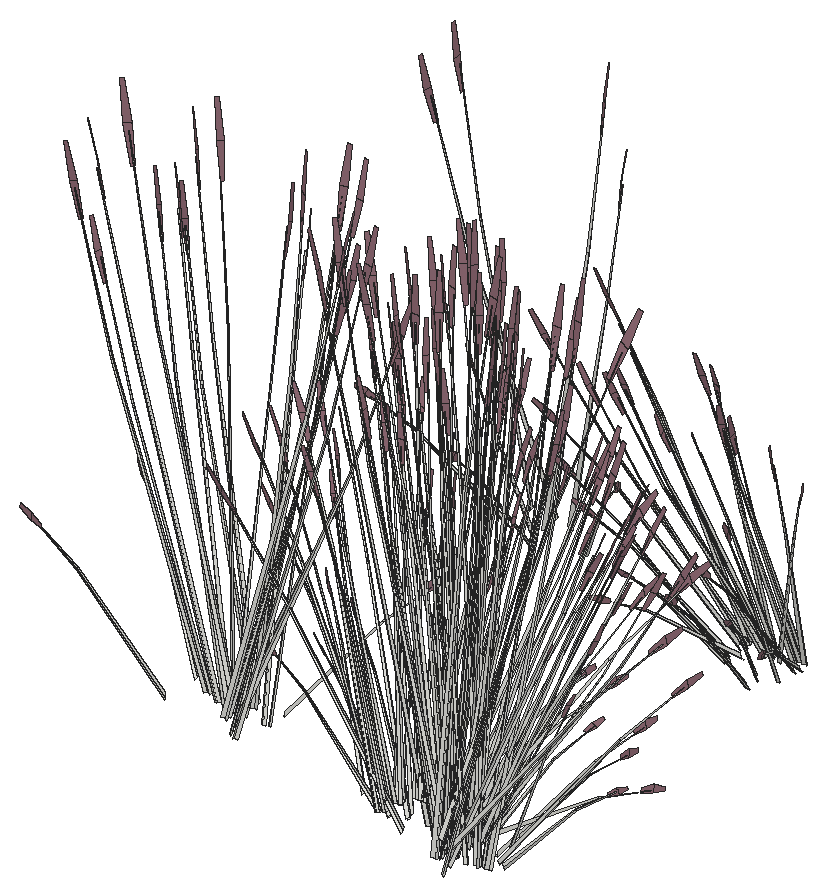
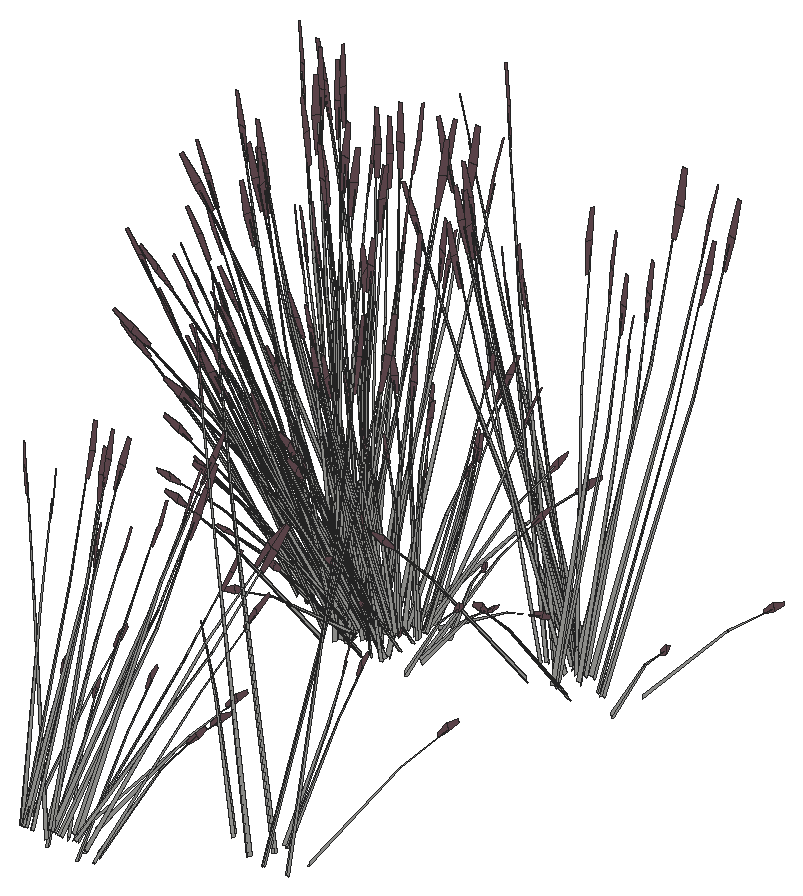
# SketchUp Ruby script. Lengths in inches.
U = 1.inch
M = Sketchup.active_model
def pt(a) = Geom::Point3d.new(a.map { |v| v * U })
def face(e, loops, mat)
  f = e.add_face(loops[0].map { |a| pt(a) })
  loops[1..].each { |l| e.add_face(l.map { |a| pt(a) }).erase! }
  f.material = f.back_material = mat if mat
  f
end
# faces: each face lists its corners as indices into pts; further lists are holes
def faces(e, pts, list, mat = nil) = list.each { |f| face(e, (f[0].is_a?(Array) ? f : [f]).map { |l| l.map { |i| pts[i] } }, mat) }
# xy, xz, yz: faces in a plane at the given z, y or x. An outline is a flat list of corners, or four numbers for a rectangle; further outlines are holes
def ring(l) = l.size == 4 ? [[l[0], l[1]], [l[2], l[1]], [l[2], l[3]], [l[0], l[3]]] : l.each_slice(2).to_a
def flat(e, list, mat, &to3) = list.each { |f| face(e, (f[0].is_a?(Array) ? f : [f]).map { |l| ring(l).map { |u, v| to3.(u, v) } }, mat) }
def xy(e, z, list, mat = nil) = flat(e, list, mat) { |x, y| [x, y, z] }
def xz(e, y, list, mat = nil) = flat(e, list, mat) { |x, z| [x, y, z] }
def yz(e, x, list, mat = nil) = flat(e, list, mat) { |y, z| [x, y, z] }
def lines(e, pts, list) = list.each { |a, b| e.add_line(pt(pts[a]), pt(pts[b])) }
# prism: a flat outline (further loops are holes) pulled along v
def prism(e, loops, v, mat = nil)
  f = face(e, loops, mat); d = Geom::Vector3d.new(v.map { |x| x * U })
  f.pushpull(f.normal.samedirection?(d) ? d.length : -d.length)
end
def box(e, o, s, mat = nil) = prism(e, [[o, [o[0] + s[0], o[1], o[2]], [o[0] + s[0], o[1] + s[1], o[2]], [o[0], o[1] + s[1], o[2]]]], [0, 0, s[2]], mat)
def at(x, y, z, deg = 0) = Geom::Transformation.translation(pt([x, y, z])) * Geom::Transformation.rotation(ORIGIN, Z_AXIS, deg.degrees)
def axes(o, x, y, z) = Geom::Transformation.new([*x, 0, *y, 0, *z, 0, *pt(o).to_a, 1])
def part(name) = M.definitions.add(name)
# library, detail: a bought-in or finely detailed component or shape, given as its bounding box
def library(name, o, s) = part(name).tap { |d| box(d.entities, o, s) }
def detail(e, o, s) = box(e.add_group.entities, o, s)
def put(e, d, t, mat = nil) = e.add_instance(d, t).tap { |i| i.material = mat if mat }
def group(e, t, mat = nil) = e.add_group.tap { |g| g.transformation = t; g.material = mat if mat }.entities
root = M.entities
M.materials.add("LightPink_Translucent").color = [144, 107, 117]
c1 = part("blade")
p = [[2.15,0.21,22],[0,0.17,0],[0.09,0.45,0],[2.18,0.31,22],[2.29,0.31,22],[0.38,0.45,0],
  [2.48,0.24,33],[2.49,0.24,33],[2.48,0.22,33]]
faces(c1.entities,p,[[0,1,2,3],[4,5,2,3],[6,3,4,7],[8,0,3,6]])
c2 = part("seeds")
p = [[0.3,-0.1,1.38],[-0.01,-0.03,1.59],[-0.01,-0.03,0.03],[0.14,-0.07,-0.07],[0.29,-0.03,3],[0.15,0.01,3.11]]
faces(c2.entities,p,[[0,1,2,3],[1,0,4,5]],"LightPink_Translucent")
c3 = part("blade with seeds")
put(c3.entities,c1,at(0,0,0))
put(c3.entities,c2,axes([2.4,0.25,30.99],[1.5799,-0.05474,1.17369],[-0.12525,1.92788,0.29478],[-0.07173,-0.02425,1.56792]))
put(root,c3,axes([43.62,594.39,43.49],[0.03108,0.16322,1.76342],[-0.62654,0.85237,-0.26939],[-0.44504,-0.04296,0.30037]))
put(root,c3,axes([78.5,593.11,40.8125],[-0.50831,0.02346,1.71376],[0.33721,-1.01661,0.13857],[0.72439,0.06288,0.73262]))
put(root,c3,axes([79.16,590.9,38.96],[0.28787,0.90242,-0.30978],[-1.14332,0.25625,0.30978],[0.23049,0.10406,1.38974]))
put(root,c3,axes([46.37,597.46,44.03],[-0.28787,-0.90242,-0.30978],[1.14332,-0.25625,0.30978],[-0.23049,-0.10406,1.38974]))
put(root,c3,axes([81.125,594.51,41.67],[0.4501,0.70615,0.0643],[-0.82077,0.34564,0.50621],[0.36181,-0.0682,0.77189]))
put(root,c3,axes([76.86,592.92,39.32],[-1.54892,-0.2182,0.49198],[0.31522,-1.23236,0.19306],[0.22636,0.119,1.70813]))
put(root,c3,axes([81.04,594.26,41.67],[-0.34623,0.9443,0.48003],[-1.13828,-0.3229,0.3958],[0.44763,-0.05675,0.9933]))
put(root,c3,axes([50.55,593.55,44.67],[1.23732,-0.68758,-0.29095],[0.8228,0.97154,-0.50002],[0.30528,0.09867,1.59708]))
put(root,c3,axes([75.62,595.96,39.14],[-0.39985,-0.89288,0],[1.1418,-0.31268,0],[0,0,1.54371]))
put(root,c3,axes([74.86,595.11,39.55],[-0.23642,0.92427,0.1448],[-1.15506,-0.16044,-0.41347],[-0.21021,-0.09491,1.26744]))
put(root,c3,axes([70.38,592.72,41.99],[1.01846,0.28891,0.35414],[-0.29705,0.84289,-0.4572],[-0.41005,0.07729,0.87481]))
put(root,c3,axes([46.05,597.85,44.02],[-1.14694,-0.51783,-0.49651],[0.68554,-0.92854,0],[-0.26122,-0.11794,1.57504]))
put(root,c3,axes([53.67,591.72,44.02],[1.14694,0.51783,-0.49651],[-0.68554,0.92854,0],[0.26122,0.11794,1.57504]))
put(root,c3,axes([77.12,595.84,39.12],[1.2866,-0.3514,-0.19198],[0.45209,1.01223,0.00008],[0.14202,-0.03884,1.73897]))
put(root,c3,axes([77.5625,596.26,39.41],[0.35402,-1.02926,0.17642],[1.29548,0.29127,0.35086],[-0.22379,0.00501,1.60407]))
put(root,c3,axes([77.27,593.92,39.15],[0.85545,0.66896,0],[-0.85545,0.66896,0],[0,0,1.69266]))
put(root,c3,axes([49.17,596.02,44.67],[-1.23732,0.68758,-0.29095],[-0.8228,-0.97154,-0.50002],[-0.30528,-0.09867,1.59708]))
put(root,c3,axes([72.41,592.67,40.28],[0.34834,-0.14982,1.77064],[0.12012,1.04605,0.13857],[-0.75452,0.1388,0.63284]))
put(root,c3,axes([79.59,593.63,39.41],[-0.96285,-0.75439,0.17642],[0.97031,-0.7317,0.35086],[-0.10634,0.15406,1.60407]))
put(root,c3,axes([77.8,592.49,38.99],[1.27479,0.1698,-0.62353],[-0.26901,1.04736,-0.16365],[0.38043,0.12691,1.37633]))
put(root,c3,axes([83.4375,594.32,39.7],[-0.75718,0.17097,1.1486],[0.35641,-0.70661,0.84392],[0.40168,0.04835,0.25299]))
put(root,c3,axes([53.35,592.11,44.03],[0.28787,0.90242,-0.30978],[-1.14332,0.25625,0.30978],[0.23049,0.10406,1.38974]))
put(root,c3,axes([75.34,596.37,39.13],[-1.23546,-0.46496,0],[0.59459,-0.96613,0],[0,0,1.62707]))
put(root,c3,axes([76.37,595.13,39.4],[-1.19666,-0.83357,-0.25192],[1.00694,-0.93603,0.5513],[-0.32224,0.09751,1.68216]))
put(root,c3,axes([73.22,596.72,39.41],[1.14694,0.51783,0.49651],[-0.68554,0.92854,0],[-0.26122,-0.11794,1.57504]))
put(root,c3,axes([77.26,593.14,39.65],[0.59459,-0.93321,0.44739],[1.23546,0.44912,-0.21531],[0,0.21512,1.43643]))
put(root,c3,axes([83.08,597.3125,41.64],[-0.11081,-0.09067,1.77383],[0.2424,-0.97188,-0.16761],[0.43649,-0.06209,0.31391]))
put(root,c3,axes([51.31,597.04,44.18],[1.2866,-0.3514,-0.19198],[0.45209,1.01223,0.00008],[0.14202,-0.03884,1.73897]))
put(root,c3,axes([68.66,593.37,41.65],[-0.20012,0.13446,1.74944],[0.01702,0.98243,-0.27667],[-0.45871,0.12776,0.14031]))
put(root,c3,axes([77.03,593.68,39.23],[0,1.19774,-0.05637],[-1.53239,0,0],[0,0.03764,1.79368]))
put(root,c3,axes([70,593.24,41.62],[-0.332,0.94205,-0.51099],[-1.13828,-0.3229,-0.3958],[-0.45829,0.08638,0.97773]))
put(root,c3,axes([69.95,592.43,41.97],[0.6166,0.93779,-0.1216],[-1.09436,0.46085,-0.67495],[-0.46117,0.12373,1.02557]))
put(root,c3,axes([77.14,592.83,39.15],[0.73619,0.86927,-0.44739],[-1.11511,0.61213,0.21531],[0.23824,0.10756,1.43643]))
put(root,c3,axes([82.12,596.5,40.86],[-0.23455,-0.87059,-0.03492],[1.10861,-0.20015,-0.15832],[0.23151,0.05519,0.52218]))
put(root,c3,axes([72.56,597.27,39.31],[-0.7662,1.03778,0],[-1.28187,-0.57875,-0.51607],[-0.29196,-0.13181,1.63711]))
put(root,c3,axes([79.25,596.48,41.97],[0.06562,-1.05324,-0.1216],[1.2424,0.02879,-0.67495],[0.4785,0.07316,1.02557]))
put(root,c3,axes([80.38,593.66,39.41],[0,-1.03566,0.49651],[1.37109,0,0],[0,0.23588,1.57504]))
put(root,c3,axes([52,593.7,44.06],[1.27479,0.1698,-0.62353],[-0.26901,1.04736,-0.16365],[0.38043,0.12691,1.37633]))
put(root,c3,axes([76.94,594.4375,39.65],[1.33077,-0.06393,0.44739],[0.12035,1.06125,-0.21531],[-0.23824,0.10756,1.43643]))
put(root,c3,axes([77.77,593.35,39.55],[1.1418,-0.30203,0.1448],[0.39985,0.86246,-0.41347],[0,0.18981,1.26744]))
put(root,c3,axes([79.06,596.0625,41.99],[-0.69728,-0.64842,0.35414],[0.79619,-0.61382,-0.4572],[0.40453,0.09339,0.87481]))
put(root,c3,axes([50.56,596.34,44.46],[-1.19666,-0.83357,-0.25192],[1.00694,-0.93603,0.5513],[-0.32224,0.09751,1.68216]))
put(root,c3,axes([75.76,594.95,39.15],[-1.33077,0.06393,-0.44739],[-0.12035,-1.06125,0.21531],[-0.23824,0.10756,1.43643]))
put(root,c3,axes([82.02,595.46,39.53],[-0.29514,-0.25472,1.43002],[0.38401,-0.84262,-0.30754],[0.59714,0.11414,0.61141]))
put(root,c3,axes([76.74,596.38,39.14],[1.23546,0.46496,0],[-0.59459,0.96613,0],[0,0,1.74954]))
put(root,c3,axes([51.33,594.04,44.21],[0.73619,0.86927,-0.44739],[-1.11511,0.61213,0.21531],[0.23824,0.10756,1.43643]))
put(root,c3,axes([80.33,595.84,41.65],[0.26289,-0.01751,1.74944],[0.72108,-0.8046,-0.27667],[0.46761,0.10621,0.14031]))
put(root,c3,axes([77.23,597.41,39.13],[-0.75665,-1.04141,-0.05142],[1.28187,-0.57875,0.51607],[-0.31588,0.09915,1.6363]))
put(root,c3,axes([76.97,594.89,39.55],[0.90538,0.62224,0.1448],[-0.75521,0.70202,-0.41347],[-0.21021,0.09491,1.26744]))
put(root,c3,axes([69.82,595.06,41.67],[-0.30393,-0.95317,0.48003],[1.19224,-0.16542,0.3958],[-0.35138,0.22417,0.9933]))
put(root,c3,axes([69.58,594.87,41.67],[-0.8413,-0.43556,0.0643],[0.48981,-0.62025,0.50621],[-0.26973,0.20053,0.77189]))
put(root,c3,axes([69.96,593.72,40.8125],[0.42521,-0.21906,1.71376],[0.35798,1.01226,0.13857],[-0.66754,0.22878,0.73262]))
put(root,c3,axes([49.95,596.16,44.21],[-1.33077,0.06393,-0.44739],[-0.12035,-1.06125,0.21531],[-0.23824,0.10756,1.43643]))
put(root,c3,axes([79.31,595.97,41.92],[1.22504,0.02494,-0.71045],[-0.08228,1.05005,0.08574],[0.51899,0.11081,1.00501]))
put(root,c3,axes([77.93,596.81,39.41],[1.14694,-0.51783,0.49651],[0.68554,0.92854,0],[-0.26122,0.11794,1.57504]))
put(root,c3,axes([76.3,595.99,39.23],[0.53281,1.18979,-0.06012],[-1.52239,0.41691,0],[0.01861,0.04155,1.72173]))
put(root,c3,axes([76.89,597.28,38.96],[-1.14332,-0.25625,-0.30978],[0.28787,-0.90242,0.30978],[-0.23049,0.10406,1.38974]))
put(root,c3,axes([68.64,595.45,39.53],[0.42589,0.08502,1.43002],[0.2745,0.86839,-0.30754],[-0.57851,0.16255,0.61141]))
put(root,c3,axes([70.55,594.74,41.99],[1.06674,-0.14801,0.35414],[0.28168,0.84611,-0.4572],[-0.30569,0.22726,0.87481]))
put(root,c3,axes([81.31,593.84,39.3125],[1.53239,0,0],[0,1.1575,-0.51607],[0,0.26363,1.63711]))
put(root,c3,axes([66.4375,594.36,41.64],[0.1564,0.02778,1.77383],[0.48382,0.91506,-0.16761],[-0.32016,0.24017,0.31391]))
put(root,c3,axes([80.7,594.43,39.13],[-1.53164,-0.00828,-0.04976],[0,-1.1575,0.49943],[-0.04813,0.2635,1.58352]))
put(root,c3,axes([77.38,593.42,39.6],[1.38012,0.49416,-0.29095],[-0.66454,1.04299,-0.50002],[0.04337,0.25608,1.59708]))
put(root,c3,axes([67.75,597.27,39.7],[0.51072,-0.46938,1.1486],[0.20153,0.74307,0.84392],[-0.36908,0.13305,0.25299]))
put(root,c3,axes([80.05,596.4,41.46],[0.69728,0.64842,-0.35414],[-0.79619,0.61382,0.4572],[0.40453,0.09339,0.87481]))
put(root,c3,axes([80.38,594.6,38.96],[-0.85545,0.64616,-0.30978],[-0.85545,-0.64616,0.30978],[0,0.20813,1.38974]))
put(root,c3,axes([76.69,594.66,39.6],[0.1428,1.18174,-0.29095],[-1.48733,0.07145,-0.50002],[-0.26191,0.15741,1.59708]))
put(root,c3,axes([79.6875,596.65,41.67],[-0.06171,0.78753,0.0643],[-0.9318,-0.02159,0.50621],[0.35694,0.08241,0.77189]))
put(root,c3,axes([77.24,594.2,39.15],[-0.59459,0.93321,-0.44739],[-1.23546,-0.44912,0.21531],[0,0.21512,1.43643]))
put(root,c3,axes([69.68,595.24,41.46],[-1.06674,0.14801,-0.35414],[-0.28168,-0.84611,0.4572],[-0.30569,0.22726,0.87481]))
put(root,c3,axes([79.77,596.4,41.67],[-0.90362,0.68241,0.48003],[-0.77932,-0.72471,0.3958],[0.42395,0.12588,0.9933]))
put(root,c3,axes([51.08,598.49,44.03],[-1.14332,-0.25625,-0.30978],[0.28787,-0.90242,0.30978],[-0.23049,0.10406,1.38974]))
put(root,c3,axes([68.125,597.14,42.58],[1.08141,0.27645,-0.06488],[-0.33265,0.85086,-0.29416],[-0.17688,0.12919,0.97024]))
put(root,c3,axes([75.8,595.57,38.99],[-0.82544,0.77843,-0.62353],[-1.0254,-0.70586,-0.16365],[-0.33076,0.19418,1.37633]))
put(root,c3,axes([51.57,594.63,44.67],[1.38012,0.49416,-0.29095],[-0.66454,1.04299,-0.50002],[0.04337,0.25608,1.59708]))
put(root,c3,axes([76.9,597.1875,41.99],[-0.18927,-0.83419,0.35414],[1.08199,-0.22027,-0.4572],[0.29062,0.23905,0.87481]))
put(root,c3,axes([77.27,596.875,39.27],[1.53422,0.33662,0.30756],[-0.38383,1.20322,-0.36492],[-0.25393,0.15059,1.64885]))
put(root,c3,axes([54.57,595.81,44.03],[-0.85545,0.64616,-0.30978],[-0.85545,-0.64616,0.30978],[0,0.20813,1.38974]))
put(root,c3,axes([77.16,597.6875,38.95],[-1.14694,0.51783,-0.49651],[-0.68554,-0.92854,0],[-0.26122,0.11794,1.57504]))
put(root,c3,axes([80.97,594.625,38.95],[0,1.03566,-0.49651],[-1.37109,0,0],[0,0.23588,1.57504]))
put(root,c3,axes([77.54,594.74,40.8125],[-0.45521,-0.17844,1.71376],[0.94204,-0.74856,0.13857],[0.58713,0.33769,0.73262]))
put(root,c3,axes([50.88,595.87,44.67],[0.1428,1.18174,-0.29095],[-1.48733,0.07145,-0.50002],[-0.26191,0.15741,1.59708]))
put(root,c3,axes([51.43,595.41,44.21],[-0.59459,0.93321,-0.44739],[-1.23546,-0.44912,0.21531],[0,0.21512,1.43643]))
put(root,c3,axes([77.63,592.39,41.41],[-1.05895,-0.53811,1.38283],[1.11816,-0.83781,0.59665],[0.34166,0.5049,1.33663]))
put(root,c3,axes([70,594.66,41.97],[1.1336,0.57106,-0.1216],[-0.65308,0.827,-0.67495],[-0.32027,0.28747,1.02557]))
put(root,c3,axes([79.23,596.77,39.7],[-0.69001,-0.29779,1.1486],[0.89096,-0.30257,0.84392],[0.24031,0.2563,0.25299]))
put(root,c3,axes([76.8,597.62,41.97],[0.73026,-0.88648,-0.1216],[1.05755,0.51071,-0.67495],[0.36761,0.25045,1.02557]))
put(root,c3,axes([71.52,594.41,40.8125],[0.30609,-0.31822,1.71376],[0.77286,0.85893,0.13857],[-0.53009,0.39116,0.73262]))
put(root,c3,axes([49.99,596.77,44.06],[-0.82544,0.77843,-0.62353],[-1.0254,-0.70586,-0.16365],[-0.33076,0.19418,1.37633]))
put(root,c3,axes([70.56,595.34,41.62],[0.31482,0.94565,-0.51099],[-1.19224,0.16542,-0.3958],[-0.34166,0.254,0.97773]))
put(root,c3,axes([71.99,596.42,41.99],[0.82919,-0.54528,0.35414],[0.78493,0.62262,-0.4572],[-0.11943,0.31634,0.87481]))
put(root,c3,axes([78.2,597.53,39.31],[0.7662,1.03778,0],[-1.28187,0.57875,-0.51607],[-0.29196,0.13181,1.63711]))
put(root,c3,axes([51.35,598.9,44.02],[-1.14694,0.51783,-0.49651],[-0.68554,-0.92854,0],[-0.26122,0.11794,1.57504]))
put(root,c3,axes([55.16,595.83,44.02],[0,1.03566,-0.49651],[-1.37109,0,0],[0,0.23588,1.57504]))
put(root,c3,axes([75.85,598.36,41.64],[0.00363,-0.12539,1.77383],[1.0502,-0.55319,-0.16761],[0.36479,0.19745,0.31391]))
put(root,c3,axes([79.42,597.88,38.43],[0.08928,-0.14952,1.76342],[1.12407,-0.44035,-0.26939],[0.34078,0.22791,0.30037]))
put(root,c3,axes([77.55,593.42,39.78],[-0.03348,-0.97511,1.41272],[1.51511,0.25277,0.59816],[-0.35835,0.53357,1.3335]))
put(root,c3,axes([77.94,594.48,39.03],[0.44936,0.94823,-0.69212],[-1.29441,0.3415,-0.18165],[0.04967,0.32109,1.52773]))
put(root,c3,axes([71.24,596.92,41.67],[-1.00708,-0.04826,0.0643],[0.02761,-0.72867,0.50621],[-0.10538,0.27912,0.77189]))
put(root,c3,axes([69.1,597.75,38.43],[0.16438,0.10347,1.76342],[0.27873,0.95868,-0.26939],[-0.36432,0.20444,0.30037]))
put(root,c3,axes([71.56,596.99,41.67],[-0.87265,-0.70663,0.48003],[0.92674,-0.60943,0.3958],[-0.16097,0.33153,0.9933]))
put(root,c3,axes([77.67,597.18,41.62],[1.20928,-0.24619,-0.51099],[0.21154,0.93233,-0.3958],[0.32481,0.26718,0.97773]))
put(root,c3,axes([74.3125,597.32,41.99],[0.36946,-0.79643,0.35414],[1.07787,0.23229,-0.4572],[0.09883,0.32066,0.87481]))
put(root,c3,axes([79.34,598.125,39.6],[-0.78586,-0.03248,1.0506],[0.51898,-0.68985,0.58006],[0.31045,0.24509,0.8241]))
put(root,c3,axes([77.07,597.95,41.67],[-0.55698,0.6579,0.0643],[-0.79316,-0.38303,0.50621],[0.25643,0.21093,0.77189]))
put(root,c3,axes([75.76,600.16,42.58],[0.84686,-0.59414,-0.06488],[0.77596,0.65071,-0.29416],[0.05463,0.18438,0.97024]))
put(root,c3,axes([77.31,597.76,41.67],[-1.21888,0.23767,0.48003],[-0.21154,-0.93233,0.3958],[0.28666,0.27478,0.9933]))
put(root,c3,axes([53.61,599.09,43.49],[0.08928,-0.14952,1.76342],[1.12407,-0.44035,-0.26939],[0.34078,0.22791,0.30037]))
put(root,c3,axes([52.125,595.69,44.09],[0.44936,0.94823,-0.69212],[-1.29441,0.3415,-0.18165],[0.04967,0.32109,1.52773]))
put(root,c3,axes([43.29,598.96,43.49],[0.16438,0.10347,1.76342],[0.27873,0.95868,-0.26939],[-0.36432,0.20444,0.30037]))
put(root,c3,axes([71.29,595.19,40.8125],[0.22818,-0.35597,1.71376],[0.95725,0.73667,0.13857],[-0.43183,0.45914,0.73262]))
put(root,c3,axes([76.77,596.45,39.53],[0.02163,-0.34331,1.43002],[1.03345,-0.38348,-0.30754],[0.31903,0.4109,0.61141]))
put(root,c3,axes([73.98,598.04,41.67],[-0.90301,0.35198,0.0643],[-0.44199,-0.64184,0.50621],[0.08721,0.28293,0.77189]))
put(root,c3,axes([71.55,597.2,41.46],[-0.82919,0.54528,-0.35414],[-0.78493,-0.62262,0.4572],[-0.11943,0.31634,0.87481]))
put(root,c3,axes([68.7,597.04,41.65],[-0.03046,0.20495,1.74944],[0.86449,0.71297,-0.27667],[-0.22632,0.33716,0.14031]))
put(root,c3,axes([71.46,596.57,42.33],[1.34686,0.05131,-0.13498],[-0.03681,0.97156,-0.74919],[-0.09356,0.37418,1.13838]))
put(root,c3,axes([73.95,597.66,41.97],[1.19922,-0.48218,-0.1216],[0.58932,0.85579,-0.67495],[0.15822,0.36063,1.02557]))
put(root,c3,axes([74.3,597.98,42],[-1.20755,-0.27075,0.53283],[0.41292,-0.89013,0.43934],[0.07257,0.35005,1.10256]))
put(root,c3,axes([72.08,599.32,39.7],[-0.03171,-0.6158,1.1486],[0.7925,0.43922,0.84392],[-0.15586,0.29352,0.25299]))
put(root,c3,axes([74.17,597.84,38.43],[0.19833,-0.05635,1.76342],[1.19302,0.31018,-0.26939],[0.03489,0.3496,0.30037]))
put(root,c3,axes([72.38,596.94,41.94],[0.87728,0.69587,-0.5672],[-0.92674,0.60943,-0.43934],[-0.13348,0.35356,1.08528]))
put(root,c3,axes([71.43,597.99,39.76],[1.11329,-0.1834,0.06507],[0.25594,0.73887,-0.86304],[-0.07058,0.37403,0.7736]))
put(root,c3,axes([74.98,597.61,41.62],[1.20468,0.25962,-0.51099],[-0.41292,0.89013,-0.3958],[0.11046,0.35838,0.97773]))
put(root,c3,axes([75.66,595.78,40.8125],[-0.28013,-0.33252,1.71376],[1.29445,-0.27994,0.13857],[0.29256,0.52202,0.73262]))
put(root,c3,axes([74.43,598.16,41.46],[-0.36946,0.79643,-0.35414],[-1.07787,-0.23229,0.4572],[0.09883,0.32066,0.87481]))
put(root,c3,axes([72.11,596.62,42.27],[-0.03189,0.95798,-0.7886],[-1.34277,-0.06434,0.09517],[-0.14171,0.40585,1.11556]))
put(root,c3,axes([48.36,599.05,43.49],[0.19833,-0.05635,1.76342],[1.19302,0.31018,-0.26939],[0.03489,0.3496,0.30037]))
put(root,c3,axes([68.6,599.14,41.64],[0.13903,-0.06253,1.77383],[1.14912,0.41591,-0.16761],[-0.027,0.34629,0.31391]))
put(root,c3,axes([73.38,595.94,40.8125],[-0.02999,-0.3975,1.71376],[1.30002,0.26369,0.13857],[-0.08041,0.56647,0.73262]))
put(root,c3,axes([74.54,597.45,41.92],[0.5849,0.8421,-0.71045],[-1.20401,0.4693,0.08574],[0.13677,0.40688,1.00501]))
put(root,c3,axes([71.16,598.77,39.53],[0.38672,-0.16338,1.43002],[0.95481,0.49262,-0.30754],[-0.28419,0.42626,0.61141]))
put(root,c3,axes([73.67,599.57,41.65],[0.15534,0.16677,1.74944],[1.25362,0.06552,-0.27667],[0.12606,0.3678,0.14031]))
put(root,c3,axes([71.66,597.97,40.3],[0.02693,-0.53464,1.54345],[1.21102,0.2824,0.21329],[-0.10493,0.5698,0.72882]))
put(root,c3,axes([52.01,637.87,43.49],[-0.20555,0.03731,1.76342],[-1.13672,-0.42002,-0.26939],[0.01907,-0.35034,0.30037]))
put(root,c3,axes([72.59,642.42,37.67],[0.28013,0.33252,1.71376],[-1.29445,0.27994,0.13857],[-0.29256,-0.52202,0.73262]))
put(root,c3,axes([74.73,640.21,38.51],[-0.18744,-0.14521,1.74944],[-1.25089,0.09206,-0.27667],[-0.19964,-0.34731,0.14031]))
put(root,c3,axes([77.625,641.9375,36.38],[-0.34835,0.20963,1.43002],[-1.04325,-0.36691,-0.30754],[0.19338,-0.4563,0.61141]))
put(root,c3,axes([76.04,642.67,38.77],[-0.5849,-0.8421,-0.71045],[1.20401,-0.4693,0.08574],[-0.13677,-0.40688,1.00501]))
put(root,c3,axes([72.23,641.54,36.38],[-0.07421,0.33879,1.43002],[-1.08488,0.28361,-0.30754],[-0.25359,-0.4379,0.61141]))
put(root,c3,axes([75.03,640.8,35.29],[-0.20555,0.03731,1.76342],[-1.13672,-0.42002,-0.26939],[0.01907,-0.35034,0.30037]))
put(root,c3,axes([48.34,639.15,43.49],[-0.11871,0.13643,1.76342],[-1.19964,0.29415,-0.26939],[-0.2898,-0.26759,0.30037]))
put(root,c3,axes([78.47,643.49,38.77],[0.03189,-0.95798,-0.71045],[1.34277,0.06434,0.08574],[0.14171,-0.40585,1.00501]))
put(root,c3,axes([50.32,642.9,44.1],[-0.50328,-1.06202,-0.69835],[1.44974,-0.38248,-0.18329],[-0.05563,-0.35963,1.54149]))
put(root,c3,axes([57.04,639.65,43.49],[-0.18342,-0.08159,1.76342],[-0.47115,-0.9115,-0.26939],[0.31784,-0.24736,0.30037]))
put(root,c3,axes([80.35,641.99,38.51],[-0.01183,-0.20612,1.74944],[-0.99913,-0.59572,-0.27667],[0.15447,-0.36112,0.14031]))
put(root,c3,axes([76.15,641.95,38.32],[0.36946,-0.79643,-0.35414],[1.07787,0.23229,0.4572],[-0.09883,-0.32066,0.87481]))
put(root,c3,axes([76.96,643,37.67],[-0.22818,0.35597,1.71376],[-0.95725,-0.73667,0.13857],[0.43183,-0.45914,0.73262]))
put(root,c3,axes([80.08,641.25,38.5],[-0.12446,0.07911,1.77383],[-1.21937,-0.26689,-0.16761],[-0.04414,-0.34521,0.31391]))
put(root,c3,axes([75.6,642.5,38.47],[-1.20468,-0.25962,-0.51099],[0.41292,-0.89013,-0.3958],[-0.11046,-0.35838,0.97773]))
put(root,c3,axes([76.34,640.27,36.56],[0.15721,0.60392,1.1486],[-0.87211,-0.33448,0.84392],[0.09385,-0.30923,0.25299]))
put(root,c3,axes([78.2,643.17,38.47],[-0.87728,-0.69587,-0.51099],[0.92674,-0.60943,-0.3958],[0.13348,-0.35356,0.97773]))
put(root,c3,axes([73.44,639.74,38.5],[-0.02286,0.12414,1.77383],[-1.12758,0.45052,-0.16761],[-0.33182,-0.23029,0.31391]))
put(root,c3,axes([51.8,638.59,44.13],[-0.84686,0.59414,-0.03893],[-0.77596,-0.65071,-0.17649],[-0.05463,-0.18438,0.58215]))
put(root,c3,axes([73.2,641.94,38.89],[1.36515,-0.26619,0.53763],[0.23692,1.04421,0.4433],[-0.32106,-0.30775,1.11249]))
put(root,c3,axes([76.28,642.14,38.53],[1.20755,0.27075,0.48003],[-0.41292,0.89013,0.3958],[-0.07257,-0.35005,0.9933]))
put(root,c3,axes([76.63,642.45,38.83],[-1.19922,0.48218,-0.1216],[-0.58932,-0.85579,-0.67495],[-0.15822,-0.36063,1.02557]))
put(root,c3,axes([79.12,643.54,38.83],[-1.34686,-0.05131,-0.1216],[0.03681,-0.97156,-0.67495],[0.09356,-0.37418,1.02557]))
put(root,c3,axes([79.03,642.91,38.32],[0.82919,-0.54528,-0.35414],[0.78493,0.62262,0.4572],[0.11943,-0.31634,0.87481]))
put(root,c3,axes([71.86,640.99,36.56],[0.63926,0.36046,1.1486],[-0.93099,0.21668,0.84392],[-0.1992,-0.27702,0.25299]))
put(root,c3,axes([76.6,642.07,38.52],[0.90301,-0.35198,0.0643],[0.44199,0.64184,0.50621],[-0.08721,-0.28293,0.77189]))
put(root,c3,axes([73.4,642.91,38.77],[-1.04497,-0.50058,-0.71045],[0.74264,-0.8772,0.08574],[-0.3786,-0.29889,1.00501]))
put(root,c3,axes([73.04,642.24,38.32],[-0.18927,-0.83419,-0.35414],[1.08199,-0.22027,0.4572],[-0.29062,-0.23905,0.87481]))
put(root,c3,axes([47.35,642.75,44.02],[0,-1.03566,-0.49651],[1.37109,0,0],[0,-0.23588,1.57504]))
put(root,c3,axes([51.16,639.68,44.02],[1.14694,-0.51783,-0.49651],[0.68554,0.92854,0],[0.26122,-0.11794,1.57504]))
put(root,c3,axes([52.52,641.81,44.06],[0.82544,-0.77843,-0.62353],[1.0254,0.70586,-0.16365],[0.33076,-0.19418,1.37633]))
